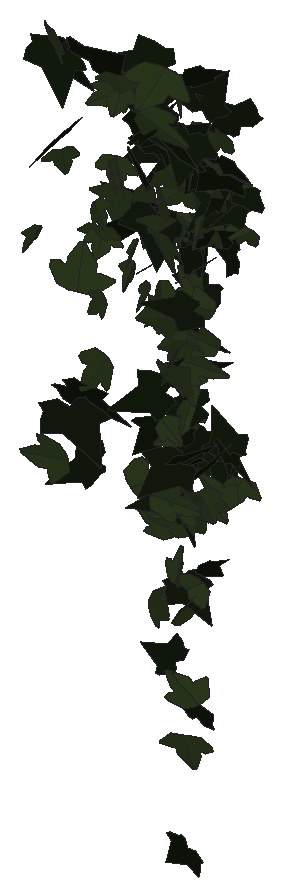
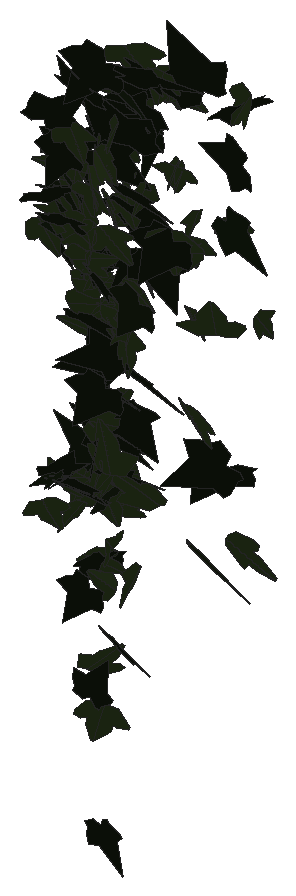
# SketchUp Ruby script. Lengths in inches.
U = 1.inch
M = Sketchup.active_model
def pt(a) = Geom::Point3d.new(a.map { |v| v * U })
def face(e, loops, mat)
  f = e.add_face(loops[0].map { |a| pt(a) })
  loops[1..].each { |l| e.add_face(l.map { |a| pt(a) }).erase! }
  f.material = f.back_material = mat if mat
  f
end
# faces: each face lists its corners as indices into pts; further lists are holes
def faces(e, pts, list, mat = nil) = list.each { |f| face(e, (f[0].is_a?(Array) ? f : [f]).map { |l| l.map { |i| pts[i] } }, mat) }
# xy, xz, yz: faces in a plane at the given z, y or x. An outline is a flat list of corners, or four numbers for a rectangle; further outlines are holes
def ring(l) = l.size == 4 ? [[l[0], l[1]], [l[2], l[1]], [l[2], l[3]], [l[0], l[3]]] : l.each_slice(2).to_a
def flat(e, list, mat, &to3) = list.each { |f| face(e, (f[0].is_a?(Array) ? f : [f]).map { |l| ring(l).map { |u, v| to3.(u, v) } }, mat) }
def xy(e, z, list, mat = nil) = flat(e, list, mat) { |x, y| [x, y, z] }
def xz(e, y, list, mat = nil) = flat(e, list, mat) { |x, z| [x, y, z] }
def yz(e, x, list, mat = nil) = flat(e, list, mat) { |y, z| [x, y, z] }
def lines(e, pts, list) = list.each { |a, b| e.add_line(pt(pts[a]), pt(pts[b])) }
# prism: a flat outline (further loops are holes) pulled along v
def prism(e, loops, v, mat = nil)
  f = face(e, loops, mat); d = Geom::Vector3d.new(v.map { |x| x * U })
  f.pushpull(f.normal.samedirection?(d) ? d.length : -d.length)
end
def box(e, o, s, mat = nil) = prism(e, [[o, [o[0] + s[0], o[1], o[2]], [o[0] + s[0], o[1] + s[1], o[2]], [o[0], o[1] + s[1], o[2]]]], [0, 0, s[2]], mat)
def at(x, y, z, deg = 0) = Geom::Transformation.translation(pt([x, y, z])) * Geom::Transformation.rotation(ORIGIN, Z_AXIS, deg.degrees)
def axes(o, x, y, z) = Geom::Transformation.new([*x, 0, *y, 0, *z, 0, *pt(o).to_a, 1])
def part(name) = M.definitions.add(name)
# library, detail: a bought-in or finely detailed component or shape, given as its bounding box
def library(name, o, s) = part(name).tap { |d| box(d.entities, o, s) }
def detail(e, o, s) = box(e.add_group.entities, o, s)
def put(e, d, t, mat = nil) = e.add_instance(d, t).tap { |i| i.material = mat if mat }
def group(e, t, mat = nil) = e.add_group.tap { |g| g.transformation = t; g.material = mat if mat }.entities
root = M.entities
M.materials.add("1026 AP 7946 SUNNY SIDE UP").color = [254, 231, 186]
M.materials.add("efeu1").color = [18, 25, 13]
M.materials.add("efeu2").color = [43, 57, 29]
c1 = part("ivyleaf_10")
p = [[0,0.5,-0.03],[-0.0625,2.02,-0.43],[-0.19,2.01,-0.46],[-0.54,1.05,-0.29],[-0.52,0.625,-0.18],[-0.83,0.76,-0.28],
  [-1.16,0.64,-0.33],[-1.15,0.33,-0.24],[-0.77,-0.39,0.02],[-0.3,-0.51,0.16],[0.04,-0.48,0.23],[-0.02,2.01,-0.4375],
  [-0.06,2.01,-0.43],[0.04,-0.49,0.23],[0.67,-0.49,0.14],[1.38,0.36,-0.2],[1.375,0.51,-0.24],[0.81,0.65,-0.19],
  [0.62,0.59,-0.15],[0.6,1.09,-0.28],[0.5,1.23,-0.31]]
faces(c1.entities,p,[[0,1,2,3,4,5,6,7,8,9,10],[11,12,0,13,14,15,16,17,18,19,20]],"efeu2")
c2 = part("ivyleaf_9")
p = [[1.54,2.16,1.25],[1.36,2.04,1.19],[-0.21,0.99,0.68],[-0.71,1.11,0.82],[-0.85,0.86,0.67],[-0.8,0.17,0.21],
  [-0.9,-0.01,0.1],[-0.67,-0.16,-0.02],[-0.08,-0.08,-0.05],[-0.03,-0.6,-0.4],[0.65,-0.88,-0.66],[0.83,-0.6,-0.49],
  [1.29,-0.42,-0.43],[1.8125,-0.07,-0.26],[1.21,0.44,0.15]]
faces(c2.entities,p,[[0,1,2,3,4,5,6,7,8,9,10,11,12,13,14]],"efeu1")
put(root,c1,axes([139.46,211.4,263.54],[-0.00046,-0.18334,0.11895],[0.02079,-0.1163,-0.18919],[0.34093,0.00684,0.0117]),"1026 AP 7946 SUNNY SIDE UP")
put(root,c1,axes([139.91,211.46,258.86],[0.17682,-0.10381,-0.30791],[-0.41832,0.13953,-0.15253],[0.26768,0.28663,-0.03497]),"1026 AP 7946 SUNNY SIDE UP")
put(root,c2,axes([139.8125,211.85,265.5625],[-0.23802,0.23885,-0.18736],[0.11756,-0.16883,-0.29135],[-0.45851,-0.16728,0.02256]),"1026 AP 7946 SUNNY SIDE UP")
put(root,c2,axes([139.33,212.12,267.03],[0.14196,-0.06783,-0.32555],[0.50761,0.02001,0.09082],[0.00161,-0.32767,0.07093]),"1026 AP 7946 SUNNY SIDE UP")
put(root,c1,axes([139.83,211.39,267.84],[-0.30835,0.26154,-0.09895],[0.07541,-0.08586,-0.33702],[-0.43239,-0.20149,0.01179]),"1026 AP 7946 SUNNY SIDE UP")
put(root,c1,axes([140.02,211.51,265.34],[-0.19199,-0.19244,-0.03232],[0.05715,0.0126,-0.23343],[0.30093,-0.12516,0.02372]),"1026 AP 7946 SUNNY SIDE UP")
put(root,c2,axes([140.02,211.31,267.61],[-0.08827,-0.33232,-0.03889],[0.0185,0.03438,-0.34696],[0.52526,-0.05706,0.00568]),"1026 AP 7946 SUNNY SIDE UP")
put(root,c2,axes([140.47,211.91,258.76],[-0.45574,0.17864,-0.01676],[-0.0002,-0.03303,-0.34974],[-0.28221,-0.28847,0.02731]),"1026 AP 7946 SUNNY SIDE UP")
put(root,c2,axes([140.2,211.53,260.4],[0.50214,0.02668,0.10234],[0.15939,-0.02956,-0.32819],[-0.02608,0.33309,-0.03535]),"1026 AP 7946 SUNNY SIDE UP")
put(root,c2,axes([140.4,211.28,260.14],[-0.10237,-0.26278,-0.23807],[0.10873,0.21922,-0.27738],[0.53782,-0.09434,0.01077]),"1026 AP 7946 SUNNY SIDE UP")
put(root,c1,axes([140.5625,211.28,262.91],[0.46672,0.17195,-0.05629],[0.04453,0.06137,0.35152],[0.28065,-0.29569,0.03783]),"1026 AP 7946 SUNNY SIDE UP")
put(root,c1,axes([140.93,211.48,261.2],[0.4103,-0.20671,-0.067],[-0.10507,0.01816,-0.34172],[0.32355,0.26802,-0.02601]),"1026 AP 7946 SUNNY SIDE UP")
put(root,c1,axes([141.21,211.8,264.74],[-0.44548,-0.11671,0.06712],[-0.066,-0.06889,-0.31239],[0.20008,-0.28258,0.0464]),"1026 AP 7946 SUNNY SIDE UP")
put(root,c2,axes([141.09,211.88,264.75],[0.4597,0.09554,-0.05856],[-0.09855,0.00771,-0.31565],[-0.14491,0.29783,0.02888]),"1026 AP 7946 SUNNY SIDE UP")
put(root,c1,axes([141.25,211.08,264.32],[-0.31551,-0.09527,0.0018],[0.00902,-0.0174,-0.22816],[0.14957,-0.19991,0.01755]),"1026 AP 7946 SUNNY SIDE UP")
put(root,c2,axes([140.87,211.29,267.67],[0.59626,-0.03494,-0.0863],[0.1357,0.02999,0.39064],[-0.0433,-0.38715,0.03575]),"1026 AP 7946 SUNNY SIDE UP")
put(root,c1,axes([141.3,211.02,262.87],[0.22014,-0.1376,-0.08951],[-0.10223,0.05666,-0.20184],[0.23387,0.15429,-0.00397]),"1026 AP 7946 SUNNY SIDE UP")
put(root,c1,axes([141.25,210.98,264.83],[0.00019,0.21631,0.07006],[-0.03419,0.06648,-0.22142],[-0.35432,-0.0063,0.0214]),"1026 AP 7946 SUNNY SIDE UP")
put(root,c1,axes([141.28,211.11,264.2],[0.24086,0.14873,-0.05869],[-0.05142,-0.04917,-0.21989],[-0.24558,0.15616,-0.01152]),"1026 AP 7946 SUNNY SIDE UP")
put(root,c2,axes([141.45,211.86,264.28],[0.06003,0.27083,-0.1476],[-0.05908,-0.14071,-0.28213],[-0.47927,0.05127,0.0163]),"1026 AP 7946 SUNNY SIDE UP")
put(root,c1,axes([141.54,211.15,267.31],[0.25625,0.03623,-0.17822],[-0.2613,-0.04956,-0.17205],[-0.09559,0.23259,-0.00744]),"1026 AP 7946 SUNNY SIDE UP")
put(root,c1,axes([141.49,211.1,265.6875],[-0.13093,0.21394,-0.0281],[0.00194,-0.03007,-0.23647],[-0.33936,-0.08271,0.00949]),"1026 AP 7946 SUNNY SIDE UP")
put(root,c2,axes([141.78,212.34,265.78],[-0.44141,0.02728,0.02365],[-0.03955,-0.02403,-0.28944],[-0.03953,-0.28062,0.02541]),"1026 AP 7946 SUNNY SIDE UP")
put(root,c1,axes([141.49,211.23,265.77],[0.35723,0.0362,0.021],[0.03086,0.00509,-0.23696],[-0.0574,0.22802,0.00333]),"1026 AP 7946 SUNNY SIDE UP")
put(root,c1,axes([141.63,211.15,267.61],[-0.36961,-0.05753,-0.01038],[0.02198,-0.01624,-0.24863],[0.08908,-0.2347,0.01829]),"1026 AP 7946 SUNNY SIDE UP")
put(root,c1,axes([141.6,211.12,265.77],[-0.16016,0.20659,0.02298],[-0.02162,0.01678,-0.23714],[-0.32583,-0.10267,0.00444]),"1026 AP 7946 SUNNY SIDE UP")
put(root,c1,axes([141.62,211.17,267.37],[0.3788,0.00369,-0.00084],[-0.00074,-0.02336,-0.24718],[-0.00591,0.23977,-0.02265]),"1026 AP 7946 SUNNY SIDE UP")
put(root,c2,axes([141.71,212.02,263.34],[0.15099,0.21868,0.18681],[0.05065,0.1805,-0.24242],[-0.44257,0.09526,0.03599]),"1026 AP 7946 SUNNY SIDE UP")
put(root,c2,axes([142.08,211.8125,267.72],[-0.3678,0.03855,0.23107],[-0.35742,-0.04725,-0.23634],[0.00845,-0.32046,0.0607]),"1026 AP 7946 SUNNY SIDE UP")
put(root,c1,axes([141.77,211.32,267.57],[-0.37834,0.03146,0.00537],[-0.01283,-0.02381,-0.24883],[-0.04842,-0.23948,0.02401]),"1026 AP 7946 SUNNY SIDE UP")
put(root,c1,axes([142.0625,212.5,264.84],[-0.33219,-0.03203,0.17819],[-0.23915,-0.1031,-0.21142],[0.13954,-0.25295,0.06187]),"1026 AP 7946 SUNNY SIDE UP")
put(root,c2,axes([141.78,211.98,264.32],[0.11022,-0.1984,-0.22544],[-0.14625,0.19742,-0.21504],[0.43944,0.11546,-0.01503]),"1026 AP 7946 SUNNY SIDE UP")
put(root,c1,axes([141.86,211.21,263.68],[-0.01403,-0.14033,0.17674],[0.11913,-0.16409,-0.13455],[0.32856,0.0535,0.05634]),"1026 AP 7946 SUNNY SIDE UP")
put(root,c1,axes([141.89,212.49,267.03],[-0.15516,0.26833,-0.05824],[0.00617,-0.06031,-0.29438],[-0.43165,-0.09732,0.01673]),"1026 AP 7946 SUNNY SIDE UP")
put(root,c1,axes([141.9,211.26,264.14],[0.15906,-0.17356,0.10405],[0.06853,-0.09255,-0.20733],[0.30903,0.10985,-0.00758]),"1026 AP 7946 SUNNY SIDE UP")
put(root,c1,axes([141.99,211.99,262.47],[-0.02092,-0.28259,-0.06023],[0.02012,0.05628,-0.29093],[0.4528,-0.01556,0.01014]),"1026 AP 7946 SUNNY SIDE UP")
put(root,c1,axes([141.94,212.05,262.86],[-0.00257,0.28054,-0.09246],[-0.02502,-0.0913,-0.2891],[-0.46324,0.00337,0.01613]),"1026 AP 7946 SUNNY SIDE UP")
put(root,c1,axes([141.98,211.47,265.32],[-0.05767,-0.19539,-0.12345],[0.10102,0.10659,-0.20054],[0.34501,-0.06387,0.03808]),"1026 AP 7946 SUNNY SIDE UP")
put(root,c2,axes([141.9375,211.54,267.7],[-0.15329,-0.07931,-0.21406],[0.33918,0.01964,-0.11211],[0.08245,-0.22827,0.06322]),"1026 AP 7946 SUNNY SIDE UP")
put(root,c2,axes([142.48,211.43,267.24],[-0.17321,-0.13566,-0.25195],[-0.26965,-0.17383,0.17845],[-0.34604,0.20335,-0.01294]),"1026 AP 7946 SUNNY SIDE UP")
put(root,c2,axes([142.21,210.94,266.15],[0.31102,-0.06706,-0.2186],[-0.31991,0.05926,-0.21471],[0.14035,0.28368,-0.00499]),"1026 AP 7946 SUNNY SIDE UP")
put(root,c1,axes([142.3125,212.6,265.625],[-0.40688,0.1,-0.04103],[-0.02015,-0.13276,-0.2548],[-0.16839,-0.22575,0.12963]),"1026 AP 7946 SUNNY SIDE UP")
put(root,c1,axes([142.29,211.13,263.39],[0.18494,-0.19113,0.0175],[-0.00044,-0.02136,-0.23102],[0.30187,0.11706,-0.01105]),"1026 AP 7946 SUNNY SIDE UP")
put(root,c2,axes([142.23,211.05,266.625],[-0.14004,0.29206,-0.02779],[-0.00091,0.02975,0.31462],[0.46143,0.08869,-0.00781]),"1026 AP 7946 SUNNY SIDE UP")
put(root,c1,axes([142.375,212.49,265.92],[0.07713,-0.25275,-0.11935],[-0.0461,0.11082,-0.26449],[0.4338,0.05671,-0.00688]),"1026 AP 7946 SUNNY SIDE UP")
put(root,c1,axes([141.97,211.4,259.07],[0.34607,-0.03886,-0.26601],[0.41016,0.02568,0.22541],[-0.00863,-0.33814,0.04567]),"1026 AP 7946 SUNNY SIDE UP")
put(root,c2,axes([142.34,212.5,263.94],[-0.33729,0.01898,-0.16296],[0.24391,-0.03639,-0.22127],[-0.05785,-0.26409,0.01719]),"1026 AP 7946 SUNNY SIDE UP")
put(root,c2,axes([142.67,211.14,261.33],[-0.47914,0.11741,0.03656],[-0.0649,-0.01054,-0.33553],[-0.18129,-0.30652,0.02349]),"1026 AP 7946 SUNNY SIDE UP")
put(root,c1,axes([142.62,212.47,264.1],[0.181,0.10334,0.24093],[-0.32773,-0.10953,0.1553],[0.2314,-0.23595,0.03149]),"1026 AP 7946 SUNNY SIDE UP")
put(root,c1,axes([142.48,212.41,264.75],[-0.28929,0.19199,0.10804],[-0.13709,0.05979,-0.27281],[-0.3146,-0.2026,0.01953]),"1026 AP 7946 SUNNY SIDE UP")
put(root,c2,axes([142.3125,211.43,264.83],[-0.35874,-0.15515,-0.18359],[0.2577,0.07285,-0.28246],[0.26619,-0.27963,0.02603]),"1026 AP 7946 SUNNY SIDE UP")
put(root,c1,axes([142.45,211.33,267.875],[0.46224,0.14148,-0.14084],[-0.17023,-0.09064,-0.33501],[-0.25937,0.31164,-0.03114]),"1026 AP 7946 SUNNY SIDE UP")
put(root,c1,axes([142.5,211.34,264.83],[-0.26822,-0.152,0.05003],[-0.03827,-0.04674,-0.23489],[0.24839,-0.17133,0.01783]),"1026 AP 7946 SUNNY SIDE UP")
put(root,c1,axes([142.35,212,259.92],[-0.49769,0.06507,0.12986],[0.19612,-0.01727,0.33269],[0.10518,0.34011,-0.00589]),"1026 AP 7946 SUNNY SIDE UP")
put(root,c2,axes([142.63,211.34,260.56],[0.12684,0.15307,-0.27062],[-0.15821,-0.24398,-0.17912],[-0.45237,0.12824,-0.01323]),"1026 AP 7946 SUNNY SIDE UP")
put(root,c2,axes([142.125,212.14,262.21],[0.39551,-0.0325,0.13791],[0.20662,-0.02837,-0.26125],[0.06599,0.28361,-0.00863]),"1026 AP 7946 SUNNY SIDE UP")
put(root,c2,axes([142.4,212.13,261.44],[0.31091,0.19064,0.04728],[0.04668,0.03377,-0.28273],[-0.30438,0.19991,0.00494]),"1026 AP 7946 SUNNY SIDE UP")
put(root,c1,axes([142.55,211.81,259.51],[-0.00193,0.0395,0.27806],[-0.14912,0.25278,-0.03711],[-0.40181,-0.094,0.01244]),"1026 AP 7946 SUNNY SIDE UP")
put(root,c1,axes([142.8,211.04,263],[-0.2028,0.0517,0.25872],[-0.40068,0.00231,-0.13545],[-0.04046,-0.28205,0.0446]),"1026 AP 7946 SUNNY SIDE UP")
put(root,c2,axes([142.61,212.5,263.02],[-0.39418,-0.06325,-0.02502],[0.04585,-0.01821,-0.26524],[0.09594,-0.25117,0.02396]),"1026 AP 7946 SUNNY SIDE UP")
put(root,c1,axes([142.54,212.01,265.98],[0.06648,-0.29743,0.08056],[0.00092,-0.08056,-0.30978],[0.48426,0.04099,-0.01047]),"1026 AP 7946 SUNNY SIDE UP")
put(root,c1,axes([142.7,211.13,265.33],[-0.07742,0.10838,-0.30289],[-0.19461,0.26737,0.12419],[0.45364,0.1332,0.00159]),"1026 AP 7946 SUNNY SIDE UP")
put(root,c2,axes([142.72,211.83,265.95],[0.03205,0.07009,-0.31294],[-0.12321,-0.2939,-0.0769],[-0.47509,0.08095,-0.00117]),"1026 AP 7946 SUNNY SIDE UP")
put(root,c2,axes([142.14,211.32,266.89],[-0.00639,-0.03281,-0.36234],[0.51093,0.13715,-0.01626],[0.21713,-0.3237,0.02759]),"1026 AP 7946 SUNNY SIDE UP")
put(root,c1,axes([142.8,211.14,258.5],[0.17924,0.1271,0.18489],[-0.23048,-0.10571,0.17311],[0.25655,-0.18377,0.02635]),"1026 AP 7946 SUNNY SIDE UP")
put(root,c2,axes([142.91,211.18,255.74],[-0.16975,0.16935,0.18404],[-0.18006,0.13694,-0.20534],[-0.34139,-0.15643,0.01679]),"1026 AP 7946 SUNNY SIDE UP")
put(root,c2,axes([142.375,211.53,266.15],[-0.2436,0.03529,0.37332],[0.49019,-0.19018,0.15535],[0.29516,0.34497,0.0501]),"1026 AP 7946 SUNNY SIDE UP")
put(root,c1,axes([142.38,211.14,267.04],[-0.23096,-0.00081,-0.27607],[0.4101,-0.07063,-0.14747],[-0.09679,-0.29731,0.03395]),"1026 AP 7946 SUNNY SIDE UP")
put(root,c1,axes([142.74,210.83,257.03],[-0.06896,0.21255,0.21867],[-0.11205,0.19977,-0.22135],[-0.45747,-0.08097,0.02125]),"1026 AP 7946 SUNNY SIDE UP")
put(root,c1,axes([142.65,211.36,265.92],[-0.18879,-0.20631,-0.14679],[0.14687,0.10841,-0.24418],[0.36475,-0.15044,0.02234]),"1026 AP 7946 SUNNY SIDE UP")
put(root,c1,axes([142.65,211.11,264.6],[-0.33274,0.15069,-0.09854],[0.10465,-0.07246,-0.26732],[-0.26119,-0.22101,0.01842]),"1026 AP 7946 SUNNY SIDE UP")
put(root,c1,axes([142.9,211.66,260.41],[0.13506,0.08951,-0.27822],[-0.29151,-0.19708,-0.12895],[-0.34035,0.20432,0.00004]),"1026 AP 7946 SUNNY SIDE UP")
put(root,c1,axes([142.72,211.2,263.08],[0.35503,-0.00157,-0.01662],[-0.02548,-0.02108,-0.23172],[0.00009,0.22538,-0.02046]),"1026 AP 7946 SUNNY SIDE UP")
put(root,c2,axes([143.03,211.32,259.12],[-0.35583,-0.0549,0.17453],[-0.24439,-0.07387,-0.23854],[0.13765,-0.27306,0.02766]),"1026 AP 7946 SUNNY SIDE UP")
put(root,c2,axes([142.83,211.86,263.76],[-0.1176,-0.12589,0.27103],[0.16469,0.24268,0.15132],[-0.4291,0.12765,-0.0162]),"1026 AP 7946 SUNNY SIDE UP")
put(root,c2,axes([142.84,211.88,259.625],[-0.0122,-0.12534,0.24066],[0.07909,0.22949,0.12952],[-0.41029,0.04796,0.01781]),"1026 AP 7946 SUNNY SIDE UP")
put(root,c2,axes([142.66,211.83,267.77],[0.34606,0.2247,0.07721],[0.0962,0.04311,-0.32348],[-0.35916,0.22805,-0.01225]),"1026 AP 7946 SUNNY SIDE UP")
put(root,c2,axes([142.96,212.45,259.54],[-0.39527,-0.0494,0.0122],[-0.01017,-0.02958,-0.26254],[0.07933,-0.24993,0.02712]),"1026 AP 7946 SUNNY SIDE UP")
put(root,c2,axes([142.98,211.23,259.89],[-0.47812,-0.03022,-0.03014],[0.0507,-0.03234,-0.31288],[0.04217,-0.30374,0.0345]),"1026 AP 7946 SUNNY SIDE UP")
put(root,c1,axes([143.12,211.42,262.38],[-0.20857,-0.00059,0.24958],[-0.37036,-0.06433,-0.13339],[0.08916,-0.26861,0.02974]),"1026 AP 7946 SUNNY SIDE UP")
put(root,c1,axes([142.86,211.8125,263.28],[-0.00926,0.27038,0.07574],[-0.00059,-0.07201,0.27818],[0.43995,0.0056,0.00197]),"1026 AP 7946 SUNNY SIDE UP")
put(root,c1,axes([142.91,211.4,264.8],[0.17006,-0.18595,-0.10197],[-0.08317,0.08251,-0.22109],[0.31982,0.12033,-0.00327]),"1026 AP 7946 SUNNY SIDE UP")
put(root,c2,axes([142.8,212.0625,257.25],[0.18816,0.20881,0.09558],[0.08955,0.07279,-0.24718],[-0.34716,0.13195,-0.01196]),"1026 AP 7946 SUNNY SIDE UP")
put(root,c1,axes([142.85,211.28,262.19],[0.2004,-0.28973,0.07596],[0.02952,-0.07403,-0.32627],[0.46982,0.12824,-0.0119]),"1026 AP 7946 SUNNY SIDE UP")
put(root,c2,axes([143.08,212.5,259.48],[-0.39615,0.0084,0.04919],[-0.07493,-0.08817,-0.24381],[0.01362,-0.24078,0.0894]),"1026 AP 7946 SUNNY SIDE UP")
put(root,c1,axes([142.81,211.07,260.74],[0.07334,0.19393,0.10964],[0.04025,0.10217,-0.20489],[-0.34467,0.0532,-0.0006]),"1026 AP 7946 SUNNY SIDE UP")
put(root,c2,axes([143.17,211.49,266.11],[-0.08713,-0.01066,-0.31238],[-0.44885,0.10613,0.05053],[0.16143,0.28934,-0.02812]),"1026 AP 7946 SUNNY SIDE UP")
put(root,c1,axes([143.08,212.23,266.46],[-0.37524,-0.00031,0.12149],[-0.1836,-0.03671,-0.24373],[0.02601,-0.26364,0.03222]),"1026 AP 7946 SUNNY SIDE UP")
put(root,c1,axes([143.1,211.35,258.8],[-0.38169,-0.06498,0.13892],[-0.19221,-0.06343,-0.25785],[0.13675,-0.27053,0.02533]),"1026 AP 7946 SUNNY SIDE UP")
put(root,c2,axes([143.09,212.68,264.91],[-0.38609,-0.05638,0.03463],[-0.04288,-0.03214,-0.25845],[0.09417,-0.24579,0.02431]),"1026 AP 7946 SUNNY SIDE UP")
put(root,c1,axes([143.22,211.14,258.75],[-0.0285,0.03755,0.25505],[-0.33832,-0.12891,0.00317],[0.20077,-0.21189,0.04154]),"1026 AP 7946 SUNNY SIDE UP")
put(root,c1,axes([142.71,212.56,264.65],[0.32889,-0.01887,0.18538],[0.27267,-0.05816,-0.21415],[0.08178,0.26979,-0.03154]),"1026 AP 7946 SUNNY SIDE UP")
put(root,c2,axes([143.12,211.88,264.27],[0.03701,-0.04069,-0.28362],[-0.3833,0.12979,-0.04051],[0.21036,0.24366,-0.02391]),"1026 AP 7946 SUNNY SIDE UP")
put(root,c2,axes([143.25,211.5,260.25],[-0.25913,0.17987,0.10692],[-0.12904,0.06388,-0.2504],[-0.29908,-0.18341,0.0154]),"1026 AP 7946 SUNNY SIDE UP")
put(root,c2,axes([143.0625,211.58,263.86],[0.03606,0.25053,0.08137],[-0.00122,0.07792,-0.25861],[-0.41238,0.02168,0.00788]),"1026 AP 7946 SUNNY SIDE UP")
put(root,c2,axes([143.27,211.46,261.12],[-0.35319,0.11192,0.09648],[-0.14996,0.01601,-0.257],[-0.17285,-0.24259,0.02583]),"1026 AP 7946 SUNNY SIDE UP")
put(root,c1,axes([143,211.1,257.6],[0.01299,0.17873,-0.21186],[0.01462,0.20646,0.18553],[0.42938,-0.01244,0.00009]),"1026 AP 7946 SUNNY SIDE UP")
put(root,c1,axes([143.02,211.52,266],[0.11391,-0.14336,-0.18862],[-0.02291,0.18777,-0.15701],[0.36391,0.0567,0.04916]),"1026 AP 7946 SUNNY SIDE UP")
put(root,c2,axes([142.77,211.4375,261.64],[0.17394,0.14223,0.3021],[0.35624,0.18789,-0.18133],[-0.36682,0.24991,-0.03285]),"1026 AP 7946 SUNNY SIDE UP")
put(root,c1,axes([143.13,211.86,264.69],[-0.37379,0.10129,0.10291],[-0.1618,0.0103,-0.26448],[-0.15355,-0.25742,0.02817]),"1026 AP 7946 SUNNY SIDE UP")
put(root,c2,axes([142.77,211.5,258.87],[0.11171,-0.24738,0.16141],[0.05903,-0.15366,-0.26599],[0.45784,0.08017,-0.00509]),"1026 AP 7946 SUNNY SIDE UP")
put(root,c1,axes([143.25,211.65,263.125],[0.0186,0.03063,0.26418],[-0.28122,-0.18397,0.03009],[0.29257,-0.17878,0.01212]),"1026 AP 7946 SUNNY SIDE UP")
put(root,c2,axes([143.17,212.53,259.7],[-0.28979,-0.15546,0.0948],[0.1028,0.0665,0.24864],[-0.26556,0.19538,-0.0072]),"1026 AP 7946 SUNNY SIDE UP")
put(root,c2,axes([143.23,211.15,251.89],[0.15541,0.00481,-0.25485],[-0.38337,-0.04366,-0.10147],[-0.06653,0.26282,-0.01061]),"1026 AP 7946 SUNNY SIDE UP")
put(root,c1,axes([142.97,211.1875,262.55],[-0.03275,-0.07097,-0.22429],[0.15038,0.1955,-0.07407],[0.3265,-0.09716,0.01162]),"1026 AP 7946 SUNNY SIDE UP")
put(root,c2,axes([143.01,211.48,266.74],[-0.36479,-0.18574,-0.11363],[0.17811,0.03144,-0.3027],[0.28824,-0.25449,0.04323]),"1026 AP 7946 SUNNY SIDE UP")
put(root,c1,axes([143.24,212,265.44],[-0.29228,0.13458,0.16252],[-0.23675,0.05662,-0.23331],[-0.22287,-0.23663,0.0347]),"1026 AP 7946 SUNNY SIDE UP")
put(root,c2,axes([142.97,211.99,267.12],[-0.28388,0.15491,0.16617],[0.19666,-0.10055,0.24444],[0.29031,0.21959,-0.0031]),"1026 AP 7946 SUNNY SIDE UP")
put(root,c1,axes([142.75,211.04,259.15],[0.06854,0.03972,0.30247],[0.36209,0.18182,-0.05954],[-0.29257,0.23433,-0.00283]),"1026 AP 7946 SUNNY SIDE UP")
put(root,c2,axes([143.36,211.15,263.33],[-0.11363,-0.11884,-0.20645],[-0.2021,-0.15382,0.1413],[-0.30446,0.14646,-0.01675]),"1026 AP 7946 SUNNY SIDE UP")
put(root,c2,axes([143.02,212.41,259.56],[-0.05767,-0.23708,0.09117],[-0.00599,-0.09025,-0.24748],[0.39861,-0.03566,0.00947]),"1026 AP 7946 SUNNY SIDE UP")
put(root,c1,axes([143.29,211.3,257.39],[0.23027,0.06101,-0.21771],[-0.29203,-0.10251,-0.16341],[-0.18629,0.2361,-0.01296]),"1026 AP 7946 SUNNY SIDE UP")
put(root,c1,axes([143.04,211.08,261.72],[-0.3828,0.05726,0.12635],[0.1966,0.00017,0.25626],[0.08033,0.27245,-0.02505]),"1026 AP 7946 SUNNY SIDE UP")
put(root,c1,axes([143.08,212.01,258.78],[0.01862,0.21739,0.1435],[0.0239,0.13737,-0.22338],[-0.40422,0.01814,-0.0066]),"1026 AP 7946 SUNNY SIDE UP")
put(root,c2,axes([142.96,211.27,259.91],[0.19496,0.21517,-0.01602],[-0.00477,0.02108,0.2556],[0.33933,-0.12333,0.0128]),"1026 AP 7946 SUNNY SIDE UP")
put(root,c1,axes([143.12,211.09,256.76],[0.0756,-0.21407,0.16791],[-0.01035,0.16581,0.22565],[-0.4241,-0.04221,0.02443]),"1026 AP 7946 SUNNY SIDE UP")
put(root,c2,axes([143.15,212.03,264.32],[-0.12484,0.23351,-0.11222],[-0.04411,0.10687,0.25461],[0.40365,0.0839,-0.00688]),"1026 AP 7946 SUNNY SIDE UP")
put(root,c1,axes([143.17,211.33,261.1],[0.11466,0.19259,-0.14282],[-0.05764,-0.1353,-0.21262],[-0.36967,0.08083,-0.01114]),"1026 AP 7946 SUNNY SIDE UP")
put(root,c2,axes([143.41,212.47,266.71],[0.08242,0.04023,0.29523],[-0.43595,-0.07568,0.06279],[0.12917,-0.2811,0.02355]),"1026 AP 7946 SUNNY SIDE UP")
put(root,c1,axes([143.51,211.47,262.51],[-0.09856,-0.03186,-0.24628],[-0.37833,-0.00581,0.06581],[-0.02162,0.2469,-0.02876]),"1026 AP 7946 SUNNY SIDE UP")
put(root,c1,axes([143.17,211.29,261.74],[0.07261,0.23258,0.0046],[0.0063,0.00241,-0.24424],[-0.36569,0.04622,-0.0033]),"1026 AP 7946 SUNNY SIDE UP")
put(root,c2,axes([143.29,211.37,254.64],[0.25011,-0.12509,0.17223],[-0.14714,0.14614,0.20436],[-0.2945,-0.17925,0.04416]),"1026 AP 7946 SUNNY SIDE UP")
put(root,c2,axes([143.1,211.28,257.44],[0.0172,-0.21807,-0.19722],[-0.02096,0.18976,-0.22381],[0.45452,0.017,-0.00286]),"1026 AP 7946 SUNNY SIDE UP")
put(root,c1,axes([143.35,211.17,255.13],[0.18386,0.22175,0.15074],[-0.13216,-0.11933,0.25702],[0.39514,-0.14309,0.01583]),"1026 AP 7946 SUNNY SIDE UP")
put(root,c2,axes([143.34,212.02,265.44],[-0.35508,0.10954,-0.17154],[0.20966,-0.10525,-0.25728],[-0.23404,-0.26048,0.02978]),"1026 AP 7946 SUNNY SIDE UP")
put(root,c2,axes([143.06,212.51,259.73],[0.22803,-0.2132,-0.02494],[-0.0054,0.02545,-0.26523],[0.33715,0.14461,0.01262]),"1026 AP 7946 SUNNY SIDE UP")
put(root,c1,axes([143.27,211.09,254.2],[-0.41452,-0.08962,-0.04134],[0.07273,-0.01356,-0.28552],[0.13583,-0.26623,0.02672]),"1026 AP 7946 SUNNY SIDE UP")
put(root,c2,axes([143.17,211.78,264.52],[0.26007,0.17271,0.09836],[0.12641,0.05341,-0.2452],[-0.28257,0.18284,-0.01917]),"1026 AP 7946 SUNNY SIDE UP")
put(root,c1,axes([143.34,212.59,258.99],[0.28315,0.14803,-0.09641],[-0.14285,-0.03719,-0.23876],[-0.23625,0.1999,0.02882]),"1026 AP 7946 SUNNY SIDE UP")
put(root,c2,axes([143.43,212.15,265.17],[-0.40725,-0.13223,0.07004],[-0.02509,-0.11243,-0.2854],[0.23299,-0.24324,0.09169]),"1026 AP 7946 SUNNY SIDE UP")
put(root,c2,axes([143.24,212.15,266.03],[0.39893,0.00408,-0.114],[-0.17203,-0.0338,-0.25985],[-0.02709,0.27473,-0.02864]),"1026 AP 7946 SUNNY SIDE UP")
put(root,c1,axes([143.18,211.37,259.02],[-0.31284,0.07939,0.16506],[0.23344,-0.05904,0.22033],[0.15557,0.24824,0.0013]),"1026 AP 7946 SUNNY SIDE UP")
put(root,c1,axes([143.52,212.48,264.5],[-0.3211,-0.01775,0.14776],[-0.22059,-0.03604,-0.21042],[0.05526,-0.24699,0.0186]),"1026 AP 7946 SUNNY SIDE UP")
put(root,c2,axes([143.48,211.86,265.04],[-0.2091,0.22931,-0.14449],[0.0789,-0.13402,-0.27301],[-0.41632,-0.14057,0.02083]),"1026 AP 7946 SUNNY SIDE UP")
put(root,c1,axes([143.29,211.5,259.2],[-0.26681,-0.2246,-0.09607],[0.14626,0.04348,-0.2859],[0.35249,-0.18805,0.04591]),"1026 AP 7946 SUNNY SIDE UP")
put(root,c1,axes([142.96,211.38,262],[-0.05543,0.02312,0.32701],[0.47919,0.09409,0.02837],[-0.14359,0.30507,-0.03156]),"1026 AP 7946 SUNNY SIDE UP")
put(root,c2,axes([143.53,211.72,265.99],[0.17668,0.15174,-0.21802],[-0.28309,-0.12253,-0.18893],[-0.29737,0.2068,0.05032]),"1026 AP 7946 SUNNY SIDE UP")
put(root,c1,axes([143.28,212.12,264.63],[0.4131,0.04786,-0.0355],[0.04545,0.03407,0.27378],[0.08112,-0.26281,0.02742]),"1026 AP 7946 SUNNY SIDE UP")
put(root,c2,axes([143.22,211.52,259.64],[0.08669,0.27386,0.05871],[-0.04508,-0.05066,0.28691],[0.43703,-0.05955,0.01795]),"1026 AP 7946 SUNNY SIDE UP")
put(root,c2,axes([143.64,212.06,264.21],[-0.08201,0.01927,-0.27101],[-0.40473,0.05539,0.05705],[0.09141,0.26251,0.00947]),"1026 AP 7946 SUNNY SIDE UP")
put(root,c1,axes([143.11,212.04,265.59],[-0.06658,-0.00738,0.26825],[0.31875,0.16481,0.03973],[-0.25735,0.20605,-0.02019]),"1026 AP 7946 SUNNY SIDE UP")
put(root,c1,axes([143.31,211.45,265.04],[0.18974,-0.15907,0.1402],[0.10963,-0.11868,-0.20592],[0.31135,0.13872,-0.01293]),"1026 AP 7946 SUNNY SIDE UP")
put(root,c1,axes([143.62,211.78,259.09],[0.25143,0.026,0.22474],[-0.34522,0.01731,0.16387],[0.00208,-0.26981,0.03057]),"1026 AP 7946 SUNNY SIDE UP")
put(root,c2,axes([143.4,212.61,265.26],[-0.23983,-0.23045,0.03615],[-0.01664,-0.03661,-0.28468],[0.36648,-0.15248,0.01073]),"1026 AP 7946 SUNNY SIDE UP")
